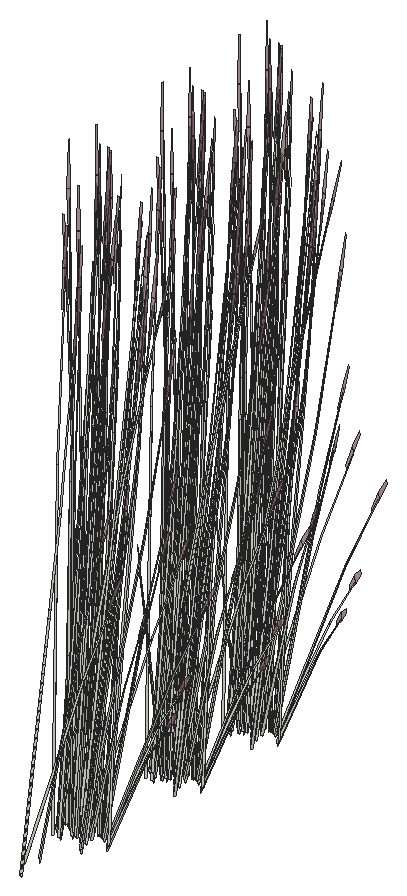
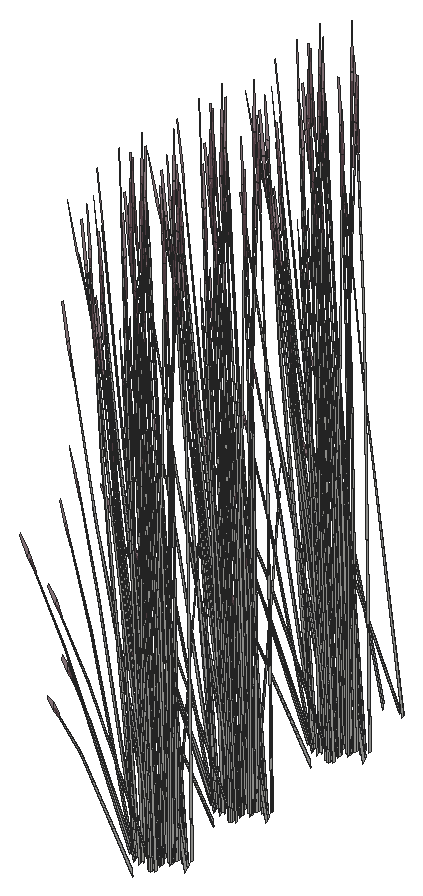
# SketchUp Ruby script. Lengths in inches.
U = 1.inch
M = Sketchup.active_model
def pt(a) = Geom::Point3d.new(a.map { |v| v * U })
def face(e, loops, mat)
  f = e.add_face(loops[0].map { |a| pt(a) })
  loops[1..].each { |l| e.add_face(l.map { |a| pt(a) }).erase! }
  f.material = f.back_material = mat if mat
  f
end
# faces: each face lists its corners as indices into pts; further lists are holes
def faces(e, pts, list, mat = nil) = list.each { |f| face(e, (f[0].is_a?(Array) ? f : [f]).map { |l| l.map { |i| pts[i] } }, mat) }
# xy, xz, yz: faces in a plane at the given z, y or x. An outline is a flat list of corners, or four numbers for a rectangle; further outlines are holes
def ring(l) = l.size == 4 ? [[l[0], l[1]], [l[2], l[1]], [l[2], l[3]], [l[0], l[3]]] : l.each_slice(2).to_a
def flat(e, list, mat, &to3) = list.each { |f| face(e, (f[0].is_a?(Array) ? f : [f]).map { |l| ring(l).map { |u, v| to3.(u, v) } }, mat) }
def xy(e, z, list, mat = nil) = flat(e, list, mat) { |x, y| [x, y, z] }
def xz(e, y, list, mat = nil) = flat(e, list, mat) { |x, z| [x, y, z] }
def yz(e, x, list, mat = nil) = flat(e, list, mat) { |y, z| [x, y, z] }
def lines(e, pts, list) = list.each { |a, b| e.add_line(pt(pts[a]), pt(pts[b])) }
# prism: a flat outline (further loops are holes) pulled along v
def prism(e, loops, v, mat = nil)
  f = face(e, loops, mat); d = Geom::Vector3d.new(v.map { |x| x * U })
  f.pushpull(f.normal.samedirection?(d) ? d.length : -d.length)
end
def box(e, o, s, mat = nil) = prism(e, [[o, [o[0] + s[0], o[1], o[2]], [o[0] + s[0], o[1] + s[1], o[2]], [o[0], o[1] + s[1], o[2]]]], [0, 0, s[2]], mat)
def at(x, y, z, deg = 0) = Geom::Transformation.translation(pt([x, y, z])) * Geom::Transformation.rotation(ORIGIN, Z_AXIS, deg.degrees)
def axes(o, x, y, z) = Geom::Transformation.new([*x, 0, *y, 0, *z, 0, *pt(o).to_a, 1])
def part(name) = M.definitions.add(name)
# library, detail: a bought-in or finely detailed component or shape, given as its bounding box
def library(name, o, s) = part(name).tap { |d| box(d.entities, o, s) }
def detail(e, o, s) = box(e.add_group.entities, o, s)
def put(e, d, t, mat = nil) = e.add_instance(d, t).tap { |i| i.material = mat if mat }
def group(e, t, mat = nil) = e.add_group.tap { |g| g.transformation = t; g.material = mat if mat }.entities
root = M.entities
M.materials.add("LightPink_Translucent").color = [144, 107, 117]
M.materials["LightPink_Translucent"].alpha = 0.75
c1 = part("blade")
p = [[2.15,0.21,22],[0,0.17,0],[0.09,0.45,0],[2.18,0.31,22],[2.29,0.31,22],[0.38,0.45,0],
  [2.48,0.24,33],[2.49,0.24,33],[2.48,0.22,33]]
faces(c1.entities,p,[[0,1,2,3],[4,5,2,3],[6,3,4,7],[8,0,3,6]])
c2 = part("seeds")
p = [[0.3,-0.1,1.38],[-0.01,-0.03,1.59],[-0.01,-0.03,0.03],[0.14,-0.07,-0.07],[0.29,-0.03,3],[0.15,0.01,3.11]]
faces(c2.entities,p,[[0,1,2,3],[1,0,4,5]],"LightPink_Translucent")
c3 = part("blade with seeds")
put(c3.entities,c1,at(0,0,0))
put(c3.entities,c2,axes([2.4,0.25,30.99],[1.5799,-0.05474,1.17369],[-0.12525,1.92788,0.29478],[-0.07173,-0.02425,1.56792]))
put(root,c3,axes([334.9,470.76,49.85],[0.18514,0.35777,-0.61156],[-0.53331,0.12885,-0.16051],[0.02046,0.12115,1.3499]))
put(root,c3,axes([335.47,472.13,50.36],[-0.32378,-0.01225,0.92831],[0.21383,-0.26028,0.51254],[0.12791,0.09247,0.72818]))
put(root,c3,axes([334.42,471.5,50.29],[0.00891,-0.12953,1.26356],[0.4258,-0.14469,-0.27174],[0.13144,0.15503,0.54024]))
put(root,c3,axes([335.77,476.65,49.32],[-0.07557,-0.03078,1.55816],[-0.19412,-0.34391,-0.23804],[0.13095,-0.09333,0.26541]))
put(root,c3,axes([332.92,476.72,50.1],[-0.31568,-0.39156,0],[0.52815,-0.21836,-0.456],[0.12029,-0.04973,1.44655]))
put(root,c3,axes([333.35,476.66,49.78],[0.47255,-0.19538,-0.43871],[0.28245,0.35034,0],[0.10763,-0.0445,1.3917]))
put(root,c3,axes([336.15,477.34,50.29],[-0.18038,-0.01157,1.26356],[-0.18479,-0.31048,-0.27174],[0.22159,-0.08783,0.54024]))
put(root,c3,axes([333.91,477.46,49.82],[0.34009,-0.2937,-0.55095],[0.42248,0.26632,-0.1446],[0.13628,-0.07327,1.21613]))
put(root,c3,axes([333.54,477.8,50.36],[-0.05884,-0.44587,-0.25709],[0.6128,-0.02696,-0.44182],[0.10791,-0.05939,1.41118]))
put(root,c3,axes([333.46,476.82,49.79],[0.47106,0.09668,-0.27372],[-0.11861,0.34048,0.27372],[0.09497,-0.03926,1.22797]))
put(root,c3,axes([333.62,478.15,50.15],[0.56891,0.18939,0.21263],[-0.2738,0.39352,0.44182],[0,-0.09071,1.41855]))
put(root,c3,axes([333.44,477.89,50.4],[-0.54829,0.02412,0.39531],[-0.04958,-0.40041,-0.19025],[0.09816,-0.04058,1.26923]))
put(root,c3,axes([335.24,476.82,50.1],[0.31568,-0.39156,0],[0.52815,0.21836,-0.456],[0.12029,0.04973,1.44655]))
put(root,c3,axes([336.49,478.37,49.75],[-0.3252,0.04689,1.25103],[-0.05176,-0.37326,0.07161],[0.22777,-0.0565,0.71188]))
put(root,c3,axes([337.08,478.04,50],[-0.31304,-0.24986,-0.05733],[0.34284,-0.22894,-0.25992],[0.09714,-0.01612,0.85731]))
put(root,c3,axes([334.21,478.07,49.95],[0,-0.45213,0],[0.63136,0,0],[0,0,1.58567]))
put(root,c3,axes([334.97,477.03,50.19],[-0.47255,-0.19538,0.43871],[0.28245,-0.35034,0],[0.10763,0.0445,1.3917]))
put(root,c3,axes([333.91,477.79,50.09],[-0.41865,0.35461,0.40429],[-0.49737,-0.31303,0.15865],[0.10093,-0.03539,1.40366]))
put(root,c3,axes([333.18,477.2,50.1875],[-0.14586,0.38834,0.15589],[-0.53375,-0.1099,0.31002],[0.0922,-0.00189,1.41735]))
put(root,c3,axes([332.96,477.52,49.41],[-0.49699,0.15644,1.13921],[-0.15819,-0.44887,0.44265],[0.30518,0.00747,1.29573]))
put(root,c3,axes([334.29,477.63,50.3125],[0.09741,-0.34873,0.12794],[0.4759,0.06053,-0.36534],[0.08661,0.03581,1.11991]))
put(root,c3,axes([336.84,478.125,49.32],[-0.02639,-0.05932,1.55816],[0.18302,-0.34702,-0.23804],[0.18462,-0.00499,0.26541]))
put(root,c3,axes([334.09,477.72,50.4],[-0.30332,-0.32798,0.39531],[0.45944,-0.23096,-0.19025],[0.09816,0.04058,1.26923]))
put(root,c3,axes([334.25,477.75,50.36],[0.50979,-0.25942,-0.25709],[0.339,0.36656,-0.44182],[0.12578,0.03723,1.41118]))
put(root,c3,axes([335.53,477.06,49.78],[0.47255,0.19538,-0.43871],[-0.28245,0.35034,0],[0.10763,0.0445,1.3917]))
put(root,c3,axes([334.63,478.17,49.95],[0.56491,0,0],[0,0.40454,0],[0,0,1.5764]))
put(root,c3,axes([334.79,477.22,50.1875],[-0.54257,0.10371,0.15589],[-0.13397,-0.38597,0.31002],[0.04839,0.05624,1.41735]))
put(root,c3,axes([335.4,477.2,49.79],[0.11861,0.34048,-0.27372],[-0.47106,0.09668,0.27372],[0.09497,0.03926,1.22797]))
put(root,c3,axes([334.45,477.97,50.1],[-0.63817,-0.08233,0.43472],[0.12987,-0.46497,0.17059],[0.09326,0.0449,1.50931]))
put(root,c3,axes([334.56,479.07,49.93],[0.53009,-0.13258,-0.16963],[0.18627,0.38191,0.00007],[0.05851,-0.01465,1.53656]))
put(root,c3,axes([334.62,478.34,49.96],[0.35245,0.2524,0],[-0.35245,0.2524,0],[0,0,1.49564]))
put(root,c3,axes([335.58,478.23,50.1875],[-0.39671,-0.28463,0.15589],[0.39978,-0.27607,0.31002],[-0.04381,0.05813,1.41735]))
put(root,c3,axes([334.84,477.8,49.82],[0.52523,0.06406,-0.55095],[-0.11084,0.39517,-0.1446],[0.15674,0.04788,1.21613]))
put(root,c3,axes([334.62,478.05,50.4],[0.24498,-0.3521,0.39531],[0.50902,0.16945,-0.19025],[0,0.08116,1.26923]))
put(root,c3,axes([334.52,478.25,50.03],[0,0.45191,-0.04981],[-0.63136,0,0],[0,0.0142,1.58489]))
put(root,c3,axes([334.57,477.93,49.95],[0.30332,0.32798,-0.39531],[-0.45944,0.23096,0.19025],[0.09816,0.04058,1.26923]))
put(root,c3,axes([335.9,478.25,50.19],[0,-0.39075,0.43871],[0.56491,0,0],[0,0.089,1.3917]))
put(root,c3,axes([334.83,478.13,50.3125],[0.47043,-0.11396,0.12794],[0.16474,0.32541,-0.36534],[0,0.07162,1.11991]))
put(root,c3,axes([336.58,478.92,50.29],[-0.1216,-0.0961,1.26356],[0.15822,-0.31792,-0.27174],[0.24603,0.04307,0.54024]))
put(root,c3,axes([334.4,479.27,49.95],[0.50902,0.17543,0],[-0.24498,0.36452,0],[0,0,1.54589]))
put(root,c3,axes([334.22,479.125,50.02],[0.21952,0.44891,-0.05313],[-0.62724,0.1573,0],[0.00767,0.01568,1.52132]))
put(root,c3,axes([336.29,478.3125,50.1],[0.63136,0,0],[0,0.43672,-0.456],[0,0.09947,1.44655]))
put(root,c3,axes([336.03,478.54,49.94],[-0.63105,-0.00312,-0.04397],[0,-0.43672,0.44129],[-0.01983,0.09942,1.3992]))
put(root,c3,axes([334.67,478.16,50.36],[0.56863,0.18645,-0.25709],[-0.2738,0.39352,-0.44182],[0.01787,0.09662,1.41118]))
put(root,c3,axes([335.9,478.6,49.79],[-0.35245,0.2438,-0.27372],[-0.35245,-0.2438,0.27372],[0,0.07853,1.22797]))
put(root,c3,axes([334.61,478.45,49.95],[-0.24498,0.3521,-0.39531],[-0.50902,-0.16945,0.19025],[0,0.08116,1.26923]))
put(root,c3,axes([336.15,478.61,49.78],[0,0.39075,-0.43871],[-0.56491,0,0],[0,0.089,1.3917]))
put(root,c3,axes([335.51,479.84,49.32],[0.03679,-0.05641,1.55816],[0.46313,-0.16615,-0.23804],[0.14041,0.08599,0.26541]))
put(root,c3,axes([334.9,478.56,49.85],[0.18514,0.35777,-0.61156],[-0.53331,0.12885,-0.16051],[0.02046,0.12115,1.3499]))
put(root,c3,axes([335.47,479.93,50.36],[-0.32378,-0.01225,0.92831],[0.21383,-0.26028,0.51254],[0.12791,0.09247,0.72818]))
put(root,c3,axes([334.42,479.3,50.29],[0.00891,-0.12953,1.26356],[0.4258,-0.14469,-0.27174],[0.13144,0.15503,0.54024]))
put(root,c3,axes([334.77,487.11,50.29],[-0.14352,0.07909,1.26356],[-0.42983,-0.13843,-0.27174],[0.07968,-0.17216,0.54024]))
put(root,c3,axes([335.77,487.35,49.32],[-0.07557,-0.03078,1.55816],[-0.19412,-0.34391,-0.23804],[0.13095,-0.09333,0.26541]))
put(root,c3,axes([332.92,487.42,50.1],[-0.31568,-0.39156,0],[0.52815,-0.21836,-0.456],[0.12029,-0.04973,1.44655]))
put(root,c3,axes([333.35,487.36,49.78],[0.47255,-0.19538,-0.43871],[0.28245,0.35034,0],[0.10763,-0.0445,1.3917]))
put(root,c3,axes([336.15,488.04,50.29],[-0.18038,-0.01157,1.26356],[-0.18479,-0.31048,-0.27174],[0.22159,-0.08783,0.54024]))
put(root,c3,axes([333.91,488.16,49.82],[0.34009,-0.2937,-0.55095],[0.42248,0.26632,-0.1446],[0.13628,-0.07327,1.21613]))
put(root,c3,axes([333.54,488.5,50.36],[-0.05884,-0.44587,-0.25709],[0.6128,-0.02696,-0.44182],[0.10791,-0.05939,1.41118]))
put(root,c3,axes([333.46,487.52,49.79],[0.47106,0.09668,-0.27372],[-0.11861,0.34048,0.27372],[0.09497,-0.03926,1.22797]))
put(root,c3,axes([333.62,488.85,50.15],[0.56891,0.18939,0.21263],[-0.2738,0.39352,0.44182],[0,-0.09071,1.41855]))
put(root,c3,axes([333.44,488.59,50.4],[-0.54829,0.02412,0.39531],[-0.04958,-0.40041,-0.19025],[0.09816,-0.04058,1.26923]))
put(root,c3,axes([335.24,487.52,50.1],[0.31568,-0.39156,0],[0.52815,0.21836,-0.456],[0.12029,0.04973,1.44655]))
put(root,c3,axes([336.49,489.07,49.75],[-0.3252,0.04689,1.25103],[-0.05176,-0.37326,0.07161],[0.22777,-0.0565,0.71188]))
put(root,c3,axes([337.08,488.74,50],[-0.31304,-0.24986,-0.05733],[0.34284,-0.22894,-0.25992],[0.09714,-0.01612,0.85731]))
put(root,c3,axes([334.21,488.77,49.95],[0,-0.45213,0],[0.63136,0,0],[0,0,1.58567]))
put(root,c3,axes([334.97,487.73,50.19],[-0.47255,-0.19538,0.43871],[0.28245,-0.35034,0],[0.10763,0.0445,1.3917]))
put(root,c3,axes([333.91,488.49,50.09],[-0.41865,0.35461,0.40429],[-0.49737,-0.31303,0.15865],[0.10093,-0.03539,1.40366]))
put(root,c3,axes([333.18,487.9,50.1875],[-0.14586,0.38834,0.15589],[-0.53375,-0.1099,0.31002],[0.0922,-0.00189,1.41735]))
put(root,c3,axes([332.96,488.21,49.41],[-0.49699,0.15644,1.13921],[-0.15819,-0.44887,0.44265],[0.30518,0.00747,1.29573]))
put(root,c3,axes([334.29,488.33,50.3125],[0.09741,-0.34873,0.12794],[0.4759,0.06053,-0.36534],[0.08661,0.03581,1.11991]))
put(root,c3,axes([336.84,488.82,49.32],[-0.02639,-0.05932,1.55816],[0.18302,-0.34702,-0.23804],[0.18462,-0.00499,0.26541]))
put(root,c3,axes([334.09,488.42,50.4],[-0.30332,-0.32798,0.39531],[0.45944,-0.23096,-0.19025],[0.09816,0.04058,1.26923]))
put(root,c3,axes([334.25,488.45,50.36],[0.50979,-0.25942,-0.25709],[0.339,0.36656,-0.44182],[0.12578,0.03723,1.41118]))
put(root,c3,axes([335.53,487.76,49.78],[0.47255,0.19538,-0.43871],[-0.28245,0.35034,0],[0.10763,0.0445,1.3917]))
put(root,c3,axes([334.63,488.87,49.95],[0.56491,0,0],[0,0.40454,0],[0,0,1.5764]))
put(root,c3,axes([334.79,487.92,50.1875],[-0.54257,0.10371,0.15589],[-0.13397,-0.38597,0.31002],[0.04839,0.05624,1.41735]))
put(root,c3,axes([335.4,487.9,49.79],[0.11861,0.34048,-0.27372],[-0.47106,0.09668,0.27372],[0.09497,0.03926,1.22797]))
put(root,c3,axes([334.45,488.67,50.1],[-0.63817,-0.08233,0.43472],[0.12987,-0.46497,0.17059],[0.09326,0.0449,1.50931]))
put(root,c3,axes([334.56,489.77,49.93],[0.53009,-0.13258,-0.16963],[0.18627,0.38191,0.00007],[0.05851,-0.01465,1.53656]))
put(root,c3,axes([334.62,489.04,49.96],[0.35245,0.2524,0],[-0.35245,0.2524,0],[0,0,1.49564]))
put(root,c3,axes([335.58,488.93,50.1875],[-0.39671,-0.28463,0.15589],[0.39978,-0.27607,0.31002],[-0.04381,0.05813,1.41735]))
put(root,c3,axes([334.84,488.5,49.82],[0.52523,0.06406,-0.55095],[-0.11084,0.39517,-0.1446],[0.15674,0.04788,1.21613]))
put(root,c3,axes([334.62,488.75,50.4],[0.24498,-0.3521,0.39531],[0.50902,0.16945,-0.19025],[0,0.08116,1.26923]))
put(root,c3,axes([334.52,488.95,50.03],[0,0.45191,-0.04981],[-0.63136,0,0],[0,0.0142,1.58489]))
put(root,c3,axes([334.57,488.63,49.95],[0.30332,0.32798,-0.39531],[-0.45944,0.23096,0.19025],[0.09816,0.04058,1.26923]))
put(root,c3,axes([335.9,488.95,50.19],[0,-0.39075,0.43871],[0.56491,0,0],[0,0.089,1.3917]))
put(root,c3,axes([334.83,488.83,50.3125],[0.47043,-0.11396,0.12794],[0.16474,0.32541,-0.36534],[0,0.07162,1.11991]))
put(root,c3,axes([336.58,489.62,50.29],[-0.1216,-0.0961,1.26356],[0.15822,-0.31792,-0.27174],[0.24603,0.04307,0.54024]))
put(root,c3,axes([334.4,489.97,49.95],[0.50902,0.17543,0],[-0.24498,0.36452,0],[0,0,1.54589]))
put(root,c3,axes([334.22,489.82,50.02],[0.21952,0.44891,-0.05313],[-0.62724,0.1573,0],[0.00767,0.01568,1.52132]))
put(root,c3,axes([336.29,489.01,50.1],[0.63136,0,0],[0,0.43672,-0.456],[0,0.09947,1.44655]))
put(root,c3,axes([336.03,489.24,49.94],[-0.63105,-0.00312,-0.04397],[0,-0.43672,0.44129],[-0.01983,0.09942,1.3992]))
put(root,c3,axes([334.67,488.86,50.36],[0.56863,0.18645,-0.25709],[-0.2738,0.39352,-0.44182],[0.01787,0.09662,1.41118]))
put(root,c3,axes([335.9,489.3,49.79],[-0.35245,0.2438,-0.27372],[-0.35245,-0.2438,0.27372],[0,0.07853,1.22797]))
put(root,c3,axes([334.61,489.15,49.95],[-0.24498,0.3521,-0.39531],[-0.50902,-0.16945,0.19025],[0,0.08116,1.26923]))
put(root,c3,axes([336.15,489.31,49.78],[0,0.39075,-0.43871],[-0.56491,0,0],[0,0.089,1.3917]))
put(root,c3,axes([335.51,490.54,49.32],[0.03679,-0.05641,1.55816],[0.46313,-0.16615,-0.23804],[0.14041,0.08599,0.26541]))
put(root,c3,axes([334.9,489.26,49.85],[0.18514,0.35777,-0.61156],[-0.53331,0.12885,-0.16051],[0.02046,0.12115,1.3499]))
put(root,c3,axes([335.47,490.63,50.36],[-0.32378,-0.01225,0.92831],[0.21383,-0.26028,0.51254],[0.12791,0.09247,0.72818]))
put(root,c3,axes([334.42,490,50.29],[0.00891,-0.12953,1.26356],[0.4258,-0.14469,-0.27174],[0.13144,0.15503,0.54024]))
put(root,c3,axes([334.77,495.88,50.29],[-0.14352,0.07909,1.26356],[-0.42983,-0.13843,-0.27174],[0.07968,-0.17216,0.54024]))
put(root,c3,axes([335.77,496.13,49.32],[-0.07557,-0.03078,1.55816],[-0.19412,-0.34391,-0.23804],[0.13095,-0.09333,0.26541]))
put(root,c3,axes([332.92,496.2,50.1],[-0.31568,-0.39156,0],[0.52815,-0.21836,-0.456],[0.12029,-0.04973,1.44655]))
put(root,c3,axes([333.35,496.14,49.78],[0.47255,-0.19538,-0.43871],[0.28245,0.35034,0],[0.10763,-0.0445,1.3917]))
put(root,c3,axes([336.15,496.8125,50.29],[-0.18038,-0.01157,1.26356],[-0.18479,-0.31048,-0.27174],[0.22159,-0.08783,0.54024]))
put(root,c3,axes([333.91,496.94,49.82],[0.34009,-0.2937,-0.55095],[0.42248,0.26632,-0.1446],[0.13628,-0.07327,1.21613]))
put(root,c3,axes([333.54,497.28,50.36],[-0.05884,-0.44587,-0.25709],[0.6128,-0.02696,-0.44182],[0.10791,-0.05939,1.41118]))
put(root,c3,axes([333.46,496.29,49.79],[0.47106,0.09668,-0.27372],[-0.11861,0.34048,0.27372],[0.09497,-0.03926,1.22797]))
put(root,c3,axes([333.62,497.63,50.15],[0.56891,0.18939,0.21263],[-0.2738,0.39352,0.44182],[0,-0.09071,1.41855]))
put(root,c3,axes([333.44,497.37,50.4],[-0.54829,0.02412,0.39531],[-0.04958,-0.40041,-0.19025],[0.09816,-0.04058,1.26923]))
put(root,c3,axes([335.24,496.3,50.1],[0.31568,-0.39156,0],[0.52815,0.21836,-0.456],[0.12029,0.04973,1.44655]))
put(root,c3,axes([336.49,497.85,49.75],[-0.3252,0.04689,1.25103],[-0.05176,-0.37326,0.07161],[0.22777,-0.0565,0.71188]))
put(root,c3,axes([337.08,497.52,50],[-0.31304,-0.24986,-0.05733],[0.34284,-0.22894,-0.25992],[0.09714,-0.01612,0.85731]))
put(root,c3,axes([334.21,497.55,49.95],[0,-0.45213,0],[0.63136,0,0],[0,0,1.58567]))
put(root,c3,axes([334.97,496.5,50.19],[-0.47255,-0.19538,0.43871],[0.28245,-0.35034,0],[0.10763,0.0445,1.3917]))
put(root,c3,axes([333.91,497.26,50.09],[-0.41865,0.35461,0.40429],[-0.49737,-0.31303,0.15865],[0.10093,-0.03539,1.40366]))
put(root,c3,axes([333.18,496.68,50.1875],[-0.14586,0.38834,0.15589],[-0.53375,-0.1099,0.31002],[0.0922,-0.00189,1.41735]))
put(root,c3,axes([332.96,496.99,49.41],[-0.49699,0.15644,1.13921],[-0.15819,-0.44887,0.44265],[0.30518,0.00747,1.29573]))
put(root,c3,axes([334.29,497.11,50.3125],[0.09741,-0.34873,0.12794],[0.4759,0.06053,-0.36534],[0.08661,0.03581,1.11991]))
put(root,c3,axes([336.84,497.6,49.32],[-0.02639,-0.05932,1.55816],[0.18302,-0.34702,-0.23804],[0.18462,-0.00499,0.26541]))
put(root,c3,axes([334.09,497.2,50.4],[-0.30332,-0.32798,0.39531],[0.45944,-0.23096,-0.19025],[0.09816,0.04058,1.26923]))
put(root,c3,axes([334.25,497.22,50.36],[0.50979,-0.25942,-0.25709],[0.339,0.36656,-0.44182],[0.12578,0.03723,1.41118]))
put(root,c3,axes([335.53,496.53,49.78],[0.47255,0.19538,-0.43871],[-0.28245,0.35034,0],[0.10763,0.0445,1.3917]))
put(root,c3,axes([334.63,497.65,49.95],[0.56491,0,0],[0,0.40454,0],[0,0,1.5764]))
put(root,c3,axes([334.79,496.7,50.1875],[-0.54257,0.10371,0.15589],[-0.13397,-0.38597,0.31002],[0.04839,0.05624,1.41735]))
put(root,c3,axes([335.4,496.68,49.79],[0.11861,0.34048,-0.27372],[-0.47106,0.09668,0.27372],[0.09497,0.03926,1.22797]))
put(root,c3,axes([334.45,497.44,50.1],[-0.63817,-0.08233,0.43472],[0.12987,-0.46497,0.17059],[0.09326,0.0449,1.50931]))
put(root,c3,axes([334.56,498.54,49.93],[0.53009,-0.13258,-0.16963],[0.18627,0.38191,0.00007],[0.05851,-0.01465,1.53656]))
put(root,c3,axes([334.62,497.82,49.96],[0.35245,0.2524,0],[-0.35245,0.2524,0],[0,0,1.49564]))
put(root,c3,axes([335.58,497.71,50.1875],[-0.39671,-0.28463,0.15589],[0.39978,-0.27607,0.31002],[-0.04381,0.05813,1.41735]))
put(root,c3,axes([334.84,497.28,49.82],[0.52523,0.06406,-0.55095],[-0.11084,0.39517,-0.1446],[0.15674,0.04788,1.21613]))
put(root,c3,axes([334.62,497.53,50.4],[0.24498,-0.3521,0.39531],[0.50902,0.16945,-0.19025],[0,0.08116,1.26923]))
put(root,c3,axes([334.52,497.73,50.03],[0,0.45191,-0.04981],[-0.63136,0,0],[0,0.0142,1.58489]))
put(root,c3,axes([334.57,497.41,49.95],[0.30332,0.32798,-0.39531],[-0.45944,0.23096,0.19025],[0.09816,0.04058,1.26923]))
put(root,c3,axes([335.9,497.72,50.19],[0,-0.39075,0.43871],[0.56491,0,0],[0,0.089,1.3917]))
put(root,c3,axes([334.83,497.61,50.3125],[0.47043,-0.11396,0.12794],[0.16474,0.32541,-0.36534],[0,0.07162,1.11991]))
put(root,c3,axes([336.58,498.4,50.29],[-0.1216,-0.0961,1.26356],[0.15822,-0.31792,-0.27174],[0.24603,0.04307,0.54024]))
put(root,c3,axes([334.4,498.75,49.95],[0.50902,0.17543,0],[-0.24498,0.36452,0],[0,0,1.54589]))
put(root,c3,axes([334.22,498.6,50.02],[0.21952,0.44891,-0.05313],[-0.62724,0.1573,0],[0.00767,0.01568,1.52132]))
put(root,c3,axes([336.29,497.79,50.1],[0.63136,0,0],[0,0.43672,-0.456],[0,0.09947,1.44655]))
put(root,c3,axes([336.03,498.01,49.94],[-0.63105,-0.00312,-0.04397],[0,-0.43672,0.44129],[-0.01983,0.09942,1.3992]))
put(root,c3,axes([334.67,497.63,50.36],[0.56863,0.18645,-0.25709],[-0.2738,0.39352,-0.44182],[0.01787,0.09662,1.41118]))
put(root,c3,axes([335.9,498.08,49.79],[-0.35245,0.2438,-0.27372],[-0.35245,-0.2438,0.27372],[0,0.07853,1.22797]))
put(root,c3,axes([334.61,497.93,49.95],[-0.24498,0.3521,-0.39531],[-0.50902,-0.16945,0.19025],[0,0.08116,1.26923]))
put(root,c3,axes([336.15,498.09,49.78],[0,0.39075,-0.43871],[-0.56491,0,0],[0,0.089,1.3917]))
put(root,c3,axes([335.51,499.3125,49.32],[0.03679,-0.05641,1.55816],[0.46313,-0.16615,-0.23804],[0.14041,0.08599,0.26541]))
put(root,c3,axes([334.9,498.03,49.85],[0.18514,0.35777,-0.61156],[-0.53331,0.12885,-0.16051],[0.02046,0.12115,1.3499]))
put(root,c3,axes([335.47,499.41,50.36],[-0.32378,-0.01225,0.92831],[0.21383,-0.26028,0.51254],[0.12791,0.09247,0.72818]))
put(root,c3,axes([334.42,498.78,50.29],[0.00891,-0.12953,1.26356],[0.4258,-0.14469,-0.27174],[0.13144,0.15503,0.54024]))
